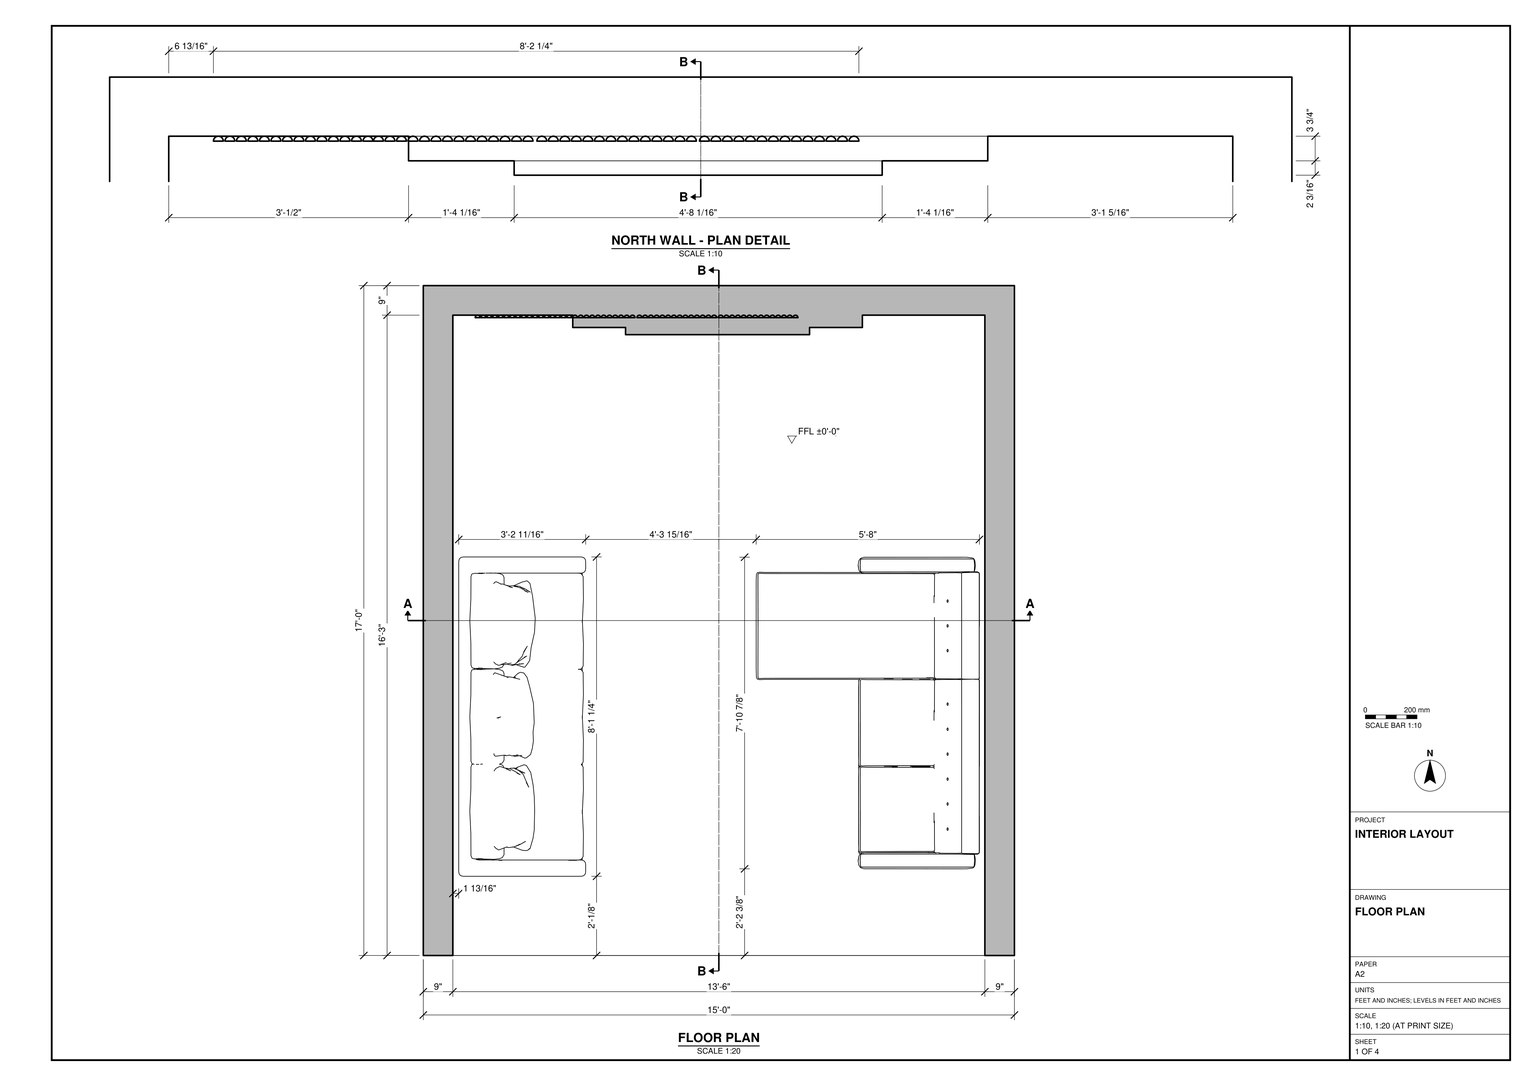
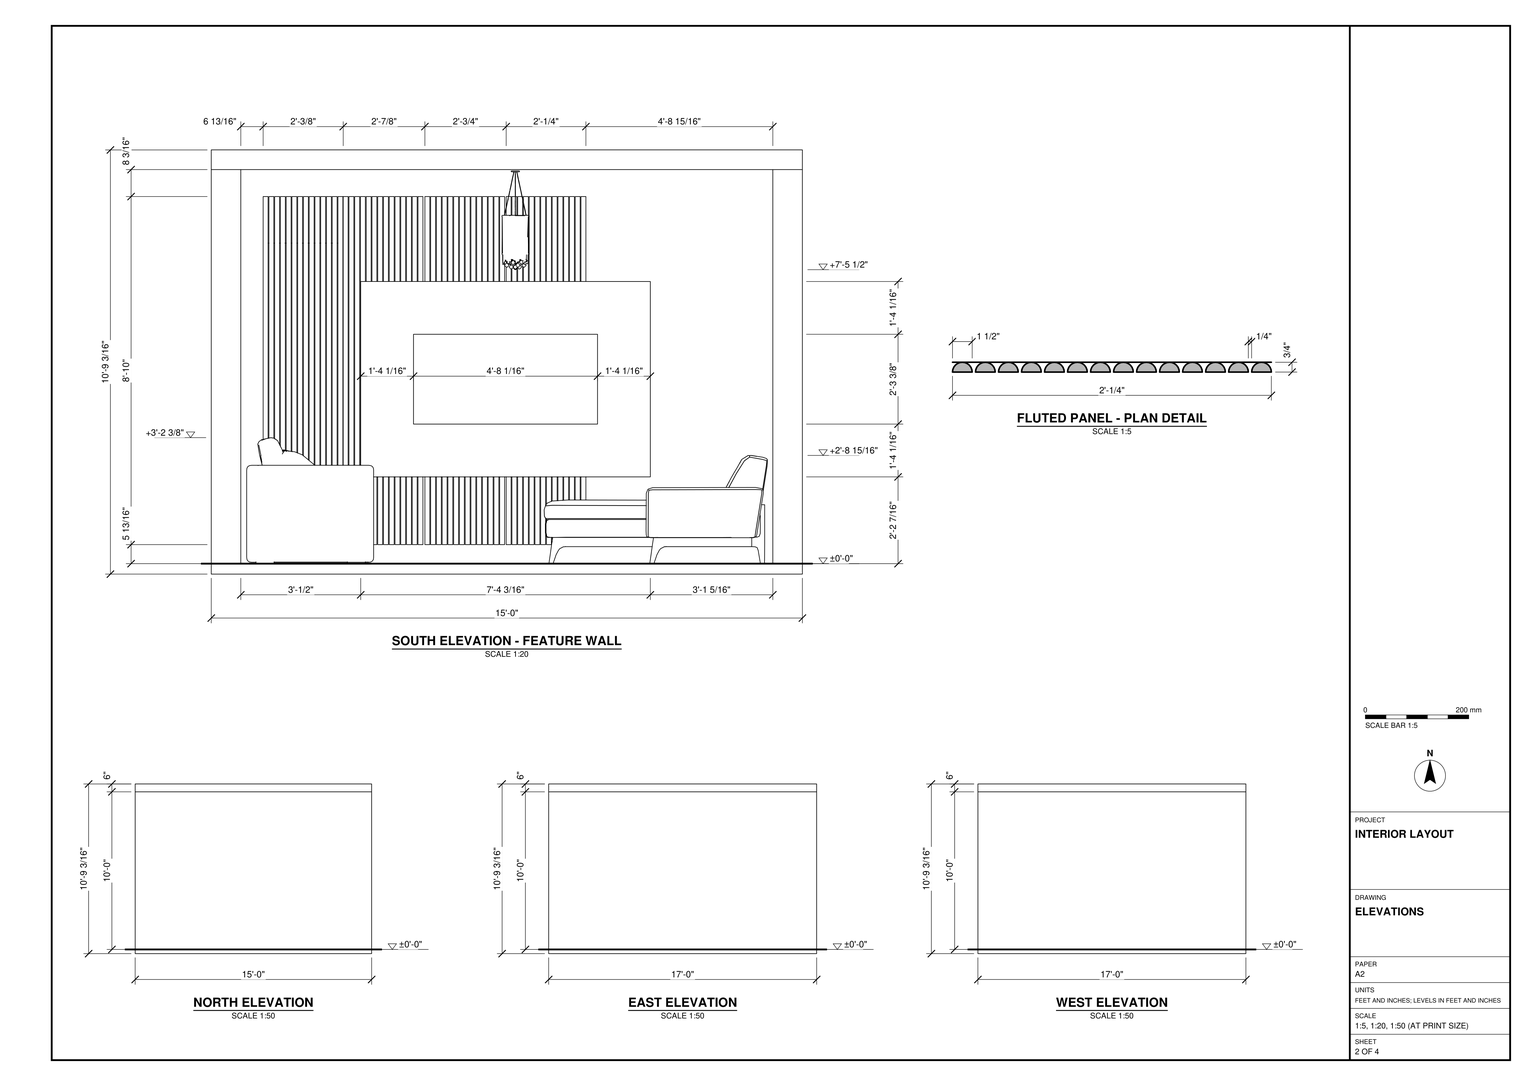
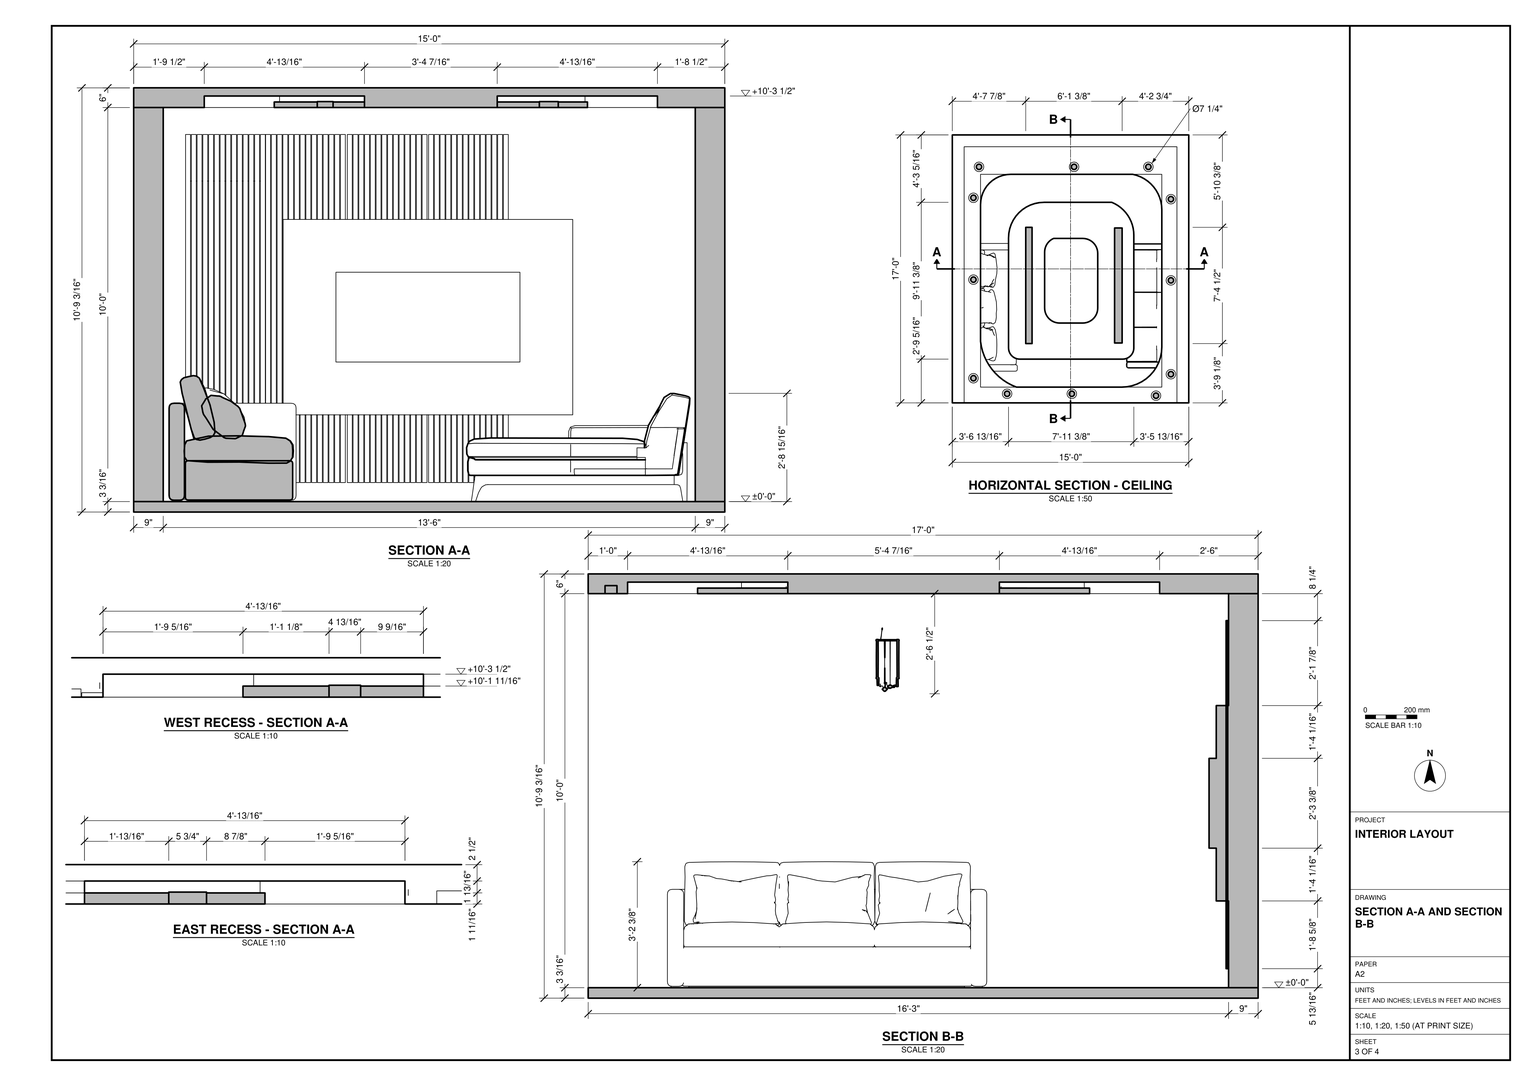
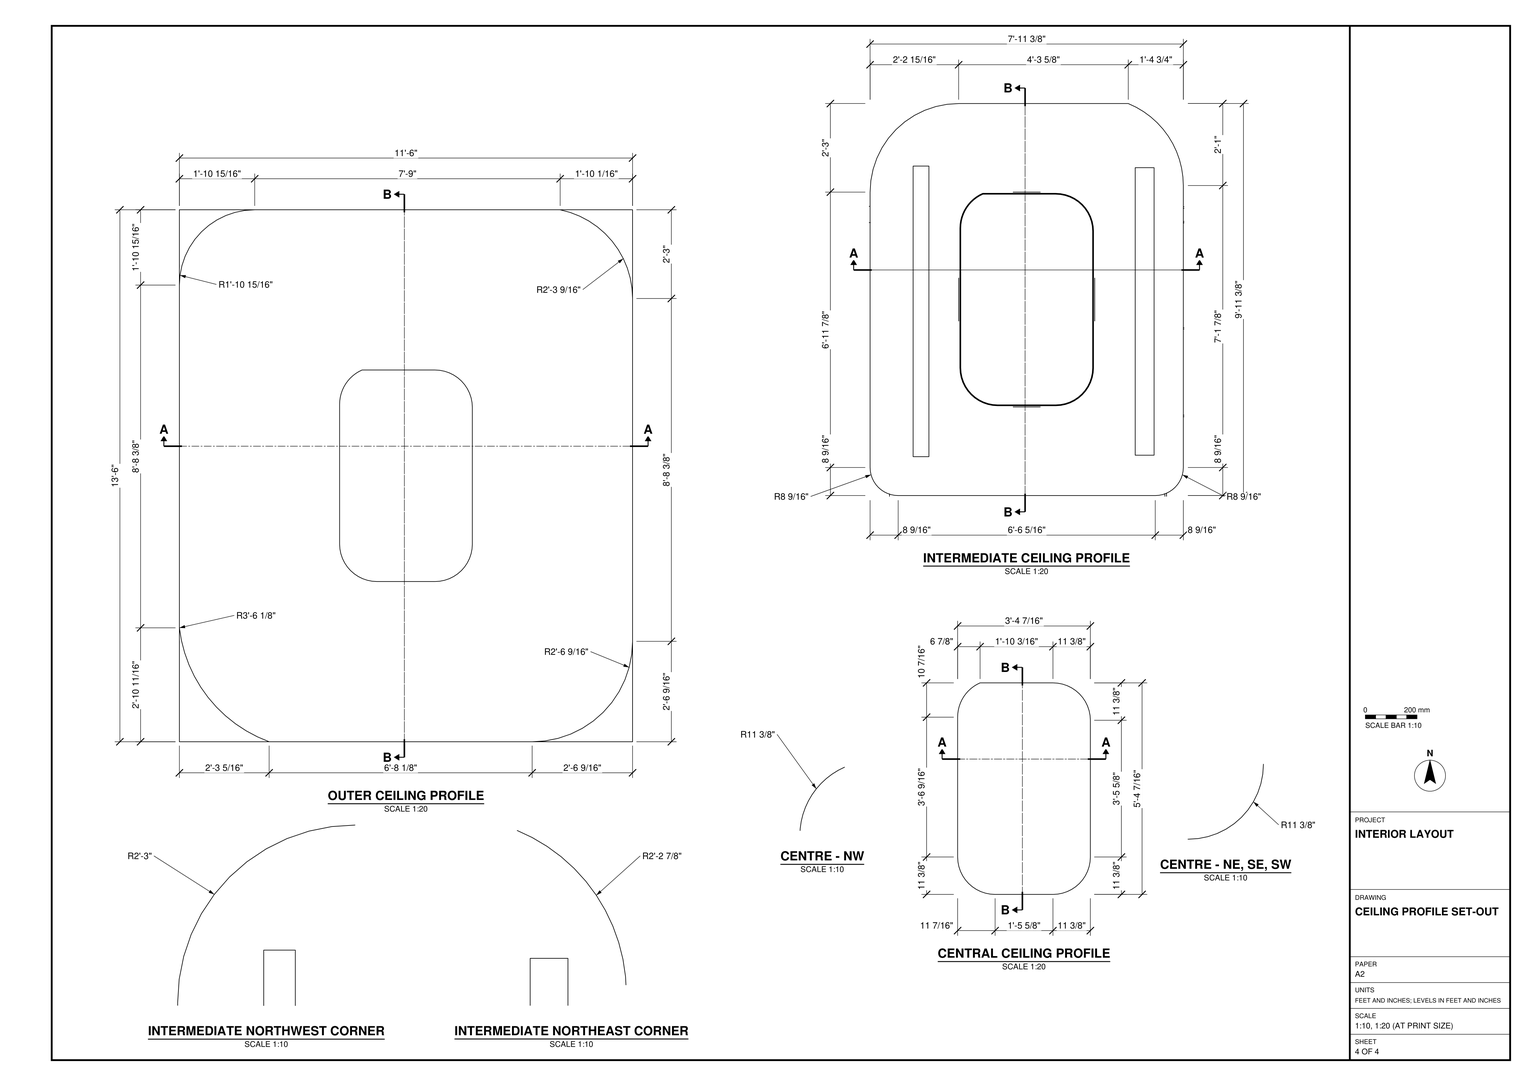
Build the sitting room in SketchUp using task_files/diagram_01.pdf. Work in feet and inches. Set the finished floor level to ±0'-0". The room shell measures 15'-0" east to west and 17'-0" north to south, with an overall height of 10'-9 3/16". Model the floor slab, the 9" north, east and west walls, and the ceiling slab. Leave the south side open as drawn.

Use the north wall plan detail and feature-wall elevation together. Form the vertical flutes with rounded profiles, then place the broad rectangular backing panel in front of them with the television centred on its face. Keep the fluted field offset to the west so it remains visible to the left of the backing panel as well as above and below it. Place the straight sofa along the west wall and the opposing sofa along the east wall, with its chaise projecting into the room at the north end. Match their footprints and setbacks to the floor plan.

Use the horizontal ceiling section for the rounded outlines, paired linear features and perimeter light positions, and the vertical sections for the recess depths and pendant position. Decor and loose items, including lights and cushions, may be any suitable library components. Keep the shell elements and each furniture or joinery piece in separate groups or components, using components for repeated parts. Save one SketchUp model as output_files/sitting_room_with_a_fluted_television_wall.skp.

# SketchUp Ruby script. Lengths in inches.
U = 1.inch
M = Sketchup.active_model
def pt(a) = Geom::Point3d.new(a.map { |v| v * U })
def face(e, loops, mat)
  f = e.add_face(loops[0].map { |a| pt(a) })
  loops[1..].each { |l| e.add_face(l.map { |a| pt(a) }).erase! }
  f.material = f.back_material = mat if mat
  f
end
# faces: each face lists its corners as indices into pts; further lists are holes
def faces(e, pts, list, mat = nil) = list.each { |f| face(e, (f[0].is_a?(Array) ? f : [f]).map { |l| l.map { |i| pts[i] } }, mat) }
# xy, xz, yz: faces in a plane at the given z, y or x. An outline is a flat list of corners, or four numbers for a rectangle; further outlines are holes
def ring(l) = l.size == 4 ? [[l[0], l[1]], [l[2], l[1]], [l[2], l[3]], [l[0], l[3]]] : l.each_slice(2).to_a
def flat(e, list, mat, &to3) = list.each { |f| face(e, (f[0].is_a?(Array) ? f : [f]).map { |l| ring(l).map { |u, v| to3.(u, v) } }, mat) }
def xy(e, z, list, mat = nil) = flat(e, list, mat) { |x, y| [x, y, z] }
def xz(e, y, list, mat = nil) = flat(e, list, mat) { |x, z| [x, y, z] }
def yz(e, x, list, mat = nil) = flat(e, list, mat) { |y, z| [x, y, z] }
def lines(e, pts, list) = list.each { |a, b| e.add_line(pt(pts[a]), pt(pts[b])) }
# prism: a flat outline (further loops are holes) pulled along v
def prism(e, loops, v, mat = nil)
  f = face(e, loops, mat); d = Geom::Vector3d.new(v.map { |x| x * U })
  f.pushpull(f.normal.samedirection?(d) ? d.length : -d.length)
end
def box(e, o, s, mat = nil) = prism(e, [[o, [o[0] + s[0], o[1], o[2]], [o[0] + s[0], o[1] + s[1], o[2]], [o[0], o[1] + s[1], o[2]]]], [0, 0, s[2]], mat)
def at(x, y, z, deg = 0) = Geom::Transformation.translation(pt([x, y, z])) * Geom::Transformation.rotation(ORIGIN, Z_AXIS, deg.degrees)
def axes(o, x, y, z) = Geom::Transformation.new([*x, 0, *y, 0, *z, 0, *pt(o).to_a, 1])
def part(name) = M.definitions.add(name)
# library, detail: a bought-in or finely detailed component or shape, given as its bounding box
def library(name, o, s) = part(name).tap { |d| box(d.entities, o, s) }
def detail(e, o, s) = box(e.add_group.entities, o, s)
def put(e, d, t, mat = nil) = e.add_instance(d, t).tap { |i| i.material = mat if mat }
def group(e, t, mat = nil) = e.add_group.tap { |g| g.transformation = t; g.material = mat if mat }.entities
root = M.entities
M.materials.add("TV").color = [52, 43, 72]
M.materials.add("[Carrera Marble]").color = [207, 207, 207]
M.materials.add("[Translucent Glass Safety]").color = [204, 235, 244]
M.materials["[Translucent Glass Safety]"].alpha = 0.5
M.materials.add("[Translucent Glass Tinted]").color = [8, 201, 241]
M.materials["[Translucent Glass Tinted]"].alpha = 0.48
M.materials.add("[Wood Veneer 01]").color = [120, 70, 37]
c1 = library("Tyler Sofa with Chaise",[-47.45,-33.89,-0.01],[94.9,67.99,32.96])
c2 = library("Sofa 193 003 01",[-48.62,-19.33,0],[97.24,38.66,38.37])
c3 = library("Recessed ceiling lights",[0,0,-4.875],[157.57,181.46,4.875])
c4 = library("Ceiling Lamp 298 001",[-7.99,-7.99,-104.37],[15.97,15.98,104.68])
c5 = library("Group\#6",[-0.5,-0.5,0],[74.38,89.5,1.8125])
c6 = library("Mesh Light\#2",[-0.5,-0.5,-0.1],[1,1,0.2])
c7 = library("Mesh Light\#1",[-0.5,-0.5,-0.1],[1,1,0.2])
c8 = part("SG_Round_Panel")
prism(c8.entities,[[[0.75,0,0],[-0.75,0,0],[-0.72,0.19,0],[-0.65,0.375,0],[-0.53,0.53,0],[-0.375,0.65,0],[-0.19,0.72,0],[0,0.75,0],[0.19,0.72,0],[0.375,0.65,0],[0.53,0.53,0],[0.65,0.375,0],[0.72,0.19,0]]],[0,0,106])
c9 = part("Group20\#1")
put(c9.entities,c8,at(17.02,195,101.6))
put(c9.entities,c8,at(18.77,195,101.6))
put(c9.entities,c8,at(20.52,195,101.6))
put(c9.entities,c8,at(22.27,195,101.6))
put(c9.entities,c8,at(24.02,195,101.6))
put(c9.entities,c8,at(25.77,195,101.6))
put(c9.entities,c8,at(27.53,195,101.6))
put(c9.entities,c8,at(29.28,195,101.6))
put(c9.entities,c8,at(31.03,195,101.6))
put(c9.entities,c8,at(32.78,195,101.6))
put(c9.entities,c8,at(34.53,195,101.6))
put(c9.entities,c8,at(36.29,195,101.6))
put(c9.entities,c8,at(38.04,195,101.6))
put(c9.entities,c8,at(39.79,195,101.6))
put(root,c1,at(135.25,73.84,0,-90))
put(root,c2,at(30.12,72.75,0,90))
g1 = group(root,at(9.49,0,89.51))
xy(g1,30.49,[[[-9.49,0,170.51,204],[12,12,150,174]],[12,12,12,46.6875,12.625,42.86,13.6,39.11,14.91,35.47,16.55,31.96,18.51,28.62,20.76,25.47,23.3,22.55,26.09,19.86,29.12,17.45,32.36,15.32,35.77,13.5,39.35,12],[119.43,12,123.42,12.26,127.34,13.04,131.125,14.33,134.71,16.1,138.04,18.32,141.04,20.96,143.68,23.96,145.9,27.29,147.67,30.875,148.96,34.66,149.74,38.58,150,42.57,150,12],[[41.86,33.3125,40.74,33.38,39.64,33.6,38.59,33.96,37.58,34.46,36.65,35.08,35.8125,35.8125,35.08,36.65,34.46,37.58,33.96,38.59,33.6,39.64,33.38,40.74,33.3125,41.86,33.3125,125.71,33.54,129.23,34.23,132.69,35.36,136.03,36.93,139.2,38.89,142.13,41.21,144.79,43.87,147.11,46.8,149.07,49.97,150.64,53.31,151.77,56.77,152.46,60.29,152.6875,111.92,152.6875,114.33,151.5625,116.61,150.21,118.75,148.63,120.73,146.85,122.52,144.89,124.11,142.76,125.48,140.48,126.62,138.08,127.52,135.58,128.17,133,128.56,130.37,128.6875,127.71,128.6875,41.86,128.62,40.74,128.4,39.64,128.04,38.59,127.54,37.58,126.92,36.65,126.1875,35.8125,125.35,35.08,124.42,34.46,123.41,33.96,122.36,33.6,121.26,33.38,120.14,33.3125],[72.19,60.79,89.81,60.79,91.3,60.89,92.76,61.18,94.18,61.66,95.51,62.32,96.42,62.92,96.75,63.14,97.875,64.125,98.86,65.25,99.68,66.49,100.34,67.82,100.82,69.24,101.11,70.7,101.21,72.19,101.21,113.81,101.11,115.3,100.82,116.76,100.34,118.18,99.68,119.51,98.86,120.75,97.875,121.875,96.75,122.86,95.51,123.68,94.18,124.34,92.76,124.82,91.3,125.11,89.81,125.21,67.62,125.21,66.63,124.72,65.7,124.14,64.83,123.47,64.02,122.72,63.29,121.9,62.65,121.01,62.09,120.06,61.63,119.0625,61.26,118.02,61,116.96,60.84,115.87,60.79,114.77,60.79,72.19,60.89,70.7,61.18,69.24,61.66,67.82,62.32,66.49,63.14,65.25,64.125,64.125,65.25,63.14,65.58,62.92,66.49,62.32,67.82,61.66,69.24,61.18,70.7,60.89],[114.04,45.6,119.79,133.16],[46.41,45.15,51.23,133.65]],[150,146.98,149.82,150.12,149.29,153.22,148.4,156.24,147.18,159.13,145.63,161.875,143.79,164.42,141.66,166.74,139.29,168.8,136.69,170.58,133.91,172.05,130.98,173.2,127.94,174,150,174],
  [12,151.0625,12,174,34.9375,174,31.94,173.8,29,173.22,26.16,172.25,23.47,170.93,20.97,169.26,18.72,167.28,16.74,165.03,15.07,162.53,13.75,159.84,12.78,157,12.2,154.06]])
xy(g1,30.49,[[72.19,60.79,70.7,60.89,69.24,61.18,67.82,61.66,66.49,62.32,65.58,62.92,65.25,63.14,64.125,64.125,63.14,65.25,62.32,66.49,61.66,67.82,61.18,69.24,60.89,70.7,60.79,72.19,60.79,114.77,60.84,115.87,61,116.96,61.26,118.02,61.63,119.0625,62.09,120.06,62.65,121.01,63.29,121.9,64.02,122.72,64.83,123.47,65.7,124.14,66.63,124.72,67.62,125.21,89.81,125.21,91.3,125.11,92.76,124.82,94.18,124.34,95.51,123.68,96.75,122.86,97.875,121.875,98.86,120.75,99.68,119.51,100.34,118.18,100.82,116.76,101.11,115.3,101.21,113.81,101.21,72.19,101.11,70.7,100.82,69.24,100.34,67.82,99.68,66.49,98.86,65.25,97.875,64.125,96.75,63.14,96.42,62.92,95.51,62.32,94.18,61.66,92.76,61.18,91.3,60.89,89.81,60.79]],"[Translucent Glass Safety]")
xy(g1,30.49,[[46.41,45.15,51.23,133.65],[114.04,45.6,119.79,133.16]],"[Translucent Glass Tinted]")
xy(g1,32.18,[[[41.86,33.3125,120.14,33.3125,121.26,33.38,122.36,33.6,123.41,33.96,124.42,34.46,125.35,35.08,126.1875,35.8125,126.92,36.65,127.54,37.58,128.04,38.59,128.4,39.64,128.62,40.74,128.6875,41.86,128.6875,127.71,128.56,130.37,128.17,133,127.52,135.58,126.62,138.08,125.48,140.48,124.11,142.76,122.52,144.89,120.73,146.85,118.75,148.63,116.61,150.21,114.33,151.5625,111.92,152.6875,60.29,152.6875,56.77,152.46,53.31,151.77,49.97,150.64,46.8,149.07,43.87,147.11,41.21,144.79,38.89,142.13,36.93,139.2,35.36,136.03,34.23,132.69,33.54,129.23,33.3125,125.71,33.3125,41.86,33.38,40.74,33.6,39.64,33.96,38.59,34.46,37.58,35.08,36.65,35.8125,35.8125,36.65,35.08,37.58,34.46,38.59,33.96,39.64,33.6,40.74,33.38],[72.19,60.79,70.7,60.89,69.24,61.18,67.82,61.66,66.49,62.32,65.58,62.92,65.25,63.14,64.125,64.125,63.14,65.25,62.32,66.49,61.66,67.82,61.18,69.24,60.89,70.7,60.79,72.19,60.79,114.77,60.84,115.87,61,116.96,61.26,118.02,61.63,119.0625,62.09,120.06,62.65,121.01,63.29,121.9,64.02,122.72,64.83,123.47,65.7,124.14,66.63,124.72,67.62,125.21,89.81,125.21,91.3,125.11,92.76,124.82,94.18,124.34,95.51,123.68,96.75,122.86,97.875,121.875,98.86,120.75,99.68,119.51,100.34,118.18,100.82,116.76,101.11,115.3,101.21,113.81,101.21,72.19,101.11,70.7,100.82,69.24,100.34,67.82,99.68,66.49,98.86,65.25,97.875,64.125,96.75,63.14,96.42,62.92,95.51,62.32,94.18,61.66,92.76,61.18,91.3,60.89,89.81,60.79],[114.04,45.6,119.79,133.16],[46.41,45.15,51.23,133.65]]])
xy(g1,33.99,[[[39.35,12,35.77,13.5,32.36,15.32,29.12,17.45,26.09,19.86,23.3,22.55,20.76,25.47,18.51,28.62,16.55,31.96,14.91,35.47,13.6,39.11,12.625,42.86,12,46.6875,12,151.0625,12.2,154.06,12.78,157,13.75,159.84,15.07,162.53,16.74,165.03,18.72,167.28,20.97,169.26,23.47,170.93,26.16,172.25,29,173.22,31.94,173.8,34.9375,174,127.94,174,130.98,173.2,133.91,172.05,136.69,170.58,139.29,168.8,141.66,166.74,143.79,164.42,145.63,161.875,147.18,159.13,148.4,156.24,149.29,153.22,149.82,150.12,150,146.98,150,42.57,149.74,38.58,148.96,34.66,147.67,30.875,145.9,27.29,143.68,23.96,141.04,20.96,138.04,18.32,134.71,16.1,131.125,14.33,127.34,13.04,123.42,12.26,119.43,12],[72.19,60.79,89.81,60.79,91.3,60.89,92.76,61.18,94.18,61.66,95.51,62.32,96.75,63.14,97.875,64.125,98.86,65.25,99.68,66.49,100.34,67.82,100.82,69.24,101.11,70.7,101.21,72.19,101.21,113.81,101.11,115.3,100.82,116.76,100.34,118.18,99.68,119.51,98.86,120.75,97.875,121.875,96.75,122.86,95.51,123.68,94.18,124.34,92.76,124.82,91.3,125.11,89.81,125.21,67.62,125.21,66.63,124.72,65.7,124.14,64.83,123.47,64.02,122.72,63.29,121.9,62.65,121.01,62.09,120.06,61.63,119.0625,61.26,118.02,61,116.96,60.84,115.87,60.79,114.77,60.79,72.19,60.89,70.7,61.18,69.24,61.66,67.82,62.32,66.49,63.14,65.25,64.125,64.125,65.25,63.14,66.49,62.32,67.82,61.66,69.24,61.18,70.7,60.89]]])
xy(g1,36.49,[[-9.49,0,170.51,204]])
xz(g1,0,[[-9.49,30.49,170.51,36.49]])
xz(g1,33.3125,[[41.86,30.49,120.14,32.18]])
xz(g1,45.15,[[46.41,30.49,51.23,32.18]])
xz(g1,45.6,[[114.04,30.49,119.79,32.18]])
xz(g1,60.79,[[72.19,30.49,89.81,32.18]])
xz(g1,125.21,[[67.62,30.49,89.81,32.18]])
xz(g1,133.16,[[114.04,30.49,119.79,32.18]])
xz(g1,133.65,[[46.41,30.49,51.23,32.18],[46.41,32.18,51.23,32.3]])
xz(g1,152.6875,[[60.29,30.49,111.92,32.18]])
xz(g1,204,[[-9.49,30.49,170.51,36.49]])
yz(g1,-9.49,[[0,30.49,204,36.49]])
yz(g1,33.3125,[[41.86,30.49,125.71,32.18]])
yz(g1,46.41,[[45.15,30.49,133.65,32.18]])
yz(g1,51.23,[[45.15,30.49,133.65,32.18]])
yz(g1,60.79,[[72.19,30.49,114.77,32.18]])
yz(g1,101.21,[[72.19,30.49,113.81,32.18]])
yz(g1,114.04,[[45.6,30.49,133.16,32.18]])
yz(g1,119.79,[[45.6,30.49,133.16,32.18]])
yz(g1,128.6875,[[41.86,30.49,127.71,32.18]])
yz(g1,170.51,[[0,30.49,204,36.49]])
p = [[40.74,33.38,30.49],[41.86,33.3125,30.49],[41.86,33.3125,32.18],[40.74,33.38,32.18],[120.14,33.3125,30.49],[121.26,33.38,30.49],
  [121.26,33.38,32.18],[120.14,33.3125,32.18],[39.64,33.6,30.49],[39.64,33.6,32.18],[122.36,33.6,30.49],[122.36,33.6,32.18],
  [38.59,33.96,30.49],[38.59,33.96,32.18],[123.41,33.96,30.49],[123.41,33.96,32.18],[37.58,34.46,30.49],[37.58,34.46,32.18],
  [124.42,34.46,30.49],[124.42,34.46,32.18],[36.65,35.08,30.49],[36.65,35.08,32.18],[125.35,35.08,30.49],[125.35,35.08,32.18],
  [35.8125,35.8125,30.49],[35.8125,35.8125,32.18],[126.1875,35.8125,30.49],[126.1875,35.8125,32.18],[35.08,36.65,30.49],[35.08,36.65,32.18],
  [126.92,36.65,30.49],[126.92,36.65,32.18],[34.46,37.58,30.49],[34.46,37.58,32.18],[127.54,37.58,30.49],[127.54,37.58,32.18],
  [33.96,38.59,30.49],[33.96,38.59,32.18],[128.04,38.59,30.49],[128.04,38.59,32.18],[33.6,39.64,30.49],[33.6,39.64,32.18],
  [128.4,39.64,30.49],[128.4,39.64,32.18],[33.38,40.74,30.49],[33.38,40.74,32.18],[128.62,40.74,30.49],[128.62,40.74,32.18],
  [33.3125,41.86,30.49],[33.3125,41.86,32.18],[128.6875,41.86,30.49],[128.6875,41.86,32.18],[72.19,60.79,30.49],[70.7,60.89,30.49],
  [70.7,60.89,32.18],[72.19,60.79,32.18],[91.3,60.89,30.49],[89.81,60.79,30.49],[89.81,60.79,32.18],[91.3,60.89,32.18],
  [69.24,61.18,30.49],[69.24,61.18,32.18],[92.76,61.18,30.49],[92.76,61.18,32.18],[67.82,61.66,30.49],[67.82,61.66,32.18],
  [94.18,61.66,30.49],[94.18,61.66,32.18],[66.49,62.32,30.49],[66.49,62.32,32.18],[95.51,62.32,30.49],[95.51,62.32,32.18],
  [65.58,62.92,30.49],[65.58,62.92,32.18],[96.42,62.92,30.49],[96.42,62.92,32.18],[65.25,63.14,30.49],[65.25,63.14,32.18],
  [96.75,63.14,30.49],[96.75,63.14,32.18],[64.125,64.125,30.49],[64.125,64.125,32.18],[97.875,64.125,30.49],[97.875,64.125,32.18],
  [63.14,65.25,30.49],[63.14,65.25,32.18],[98.86,65.25,30.49],[98.86,65.25,32.18],[62.32,66.49,30.49],[62.32,66.49,32.18],
  [99.68,66.49,30.49],[99.68,66.49,32.18],[61.66,67.82,30.49],[61.66,67.82,32.18],[100.34,67.82,30.49],[100.34,67.82,32.18],
  [61.18,69.24,30.49],[61.18,69.24,32.18],[100.82,69.24,30.49],[100.82,69.24,32.18],[60.89,70.7,30.49],[60.89,70.7,32.18],
  [101.11,70.7,30.49],[101.11,70.7,32.18],[60.79,72.19,30.49],[60.79,72.19,32.18],[101.21,72.19,30.49],[101.21,72.19,32.18],
  [101.11,115.3,30.49],[101.21,113.81,30.49],[101.21,113.81,32.18],[101.11,115.3,32.18],[60.79,114.77,30.49],[60.84,115.87,30.49],
  [60.84,115.87,32.18],[60.79,114.77,32.18],[100.82,116.76,30.49],[100.82,116.76,32.18],[61,116.96,30.49],[61,116.96,32.18],
  [100.34,118.18,30.49],[100.34,118.18,32.18],[61.26,118.02,30.49],[61.26,118.02,32.18],[61.63,119.0625,30.49],[61.63,119.0625,32.18],
  [99.68,119.51,30.49],[99.68,119.51,32.18],[62.09,120.06,30.49],[62.09,120.06,32.18],[98.86,120.75,30.49],[98.86,120.75,32.18],
  [62.65,121.01,30.49],[62.65,121.01,32.18],[97.875,121.875,30.49],[97.875,121.875,32.18],[63.29,121.9,30.49],[63.29,121.9,32.18],
  [64.02,122.72,30.49],[64.02,122.72,32.18],[96.75,122.86,30.49],[96.75,122.86,32.18],[64.83,123.47,30.49],[64.83,123.47,32.18],
  [95.51,123.68,30.49],[95.51,123.68,32.18],[65.7,124.14,30.49],[65.7,124.14,32.18],[94.18,124.34,30.49],[94.18,124.34,32.18],
  [66.63,124.72,30.49],[66.63,124.72,32.18],[92.76,124.82,30.49],[92.76,124.82,32.18],[67.62,125.21,30.49],[67.62,125.21,32.18],
  [91.3,125.11,30.49],[91.3,125.11,32.18],[89.81,125.21,30.49],[89.81,125.21,32.18],[33.54,129.23,30.49],[33.3125,125.71,30.49],
  [33.3125,125.71,32.18],[33.54,129.23,32.18],[128.6875,127.71,30.49],[128.56,130.37,30.49],[128.56,130.37,32.18],[128.6875,127.71,32.18],
  [34.23,132.69,30.49],[34.23,132.69,32.18],[128.17,133,30.49],[128.17,133,32.18],[35.36,136.03,30.49],[35.36,136.03,32.18],
  [127.52,135.58,30.49],[127.52,135.58,32.18],[126.62,138.08,30.49],[126.62,138.08,32.18],[36.93,139.2,30.49],[36.93,139.2,32.18],
  [125.48,140.48,30.49],[125.48,140.48,32.18],[38.89,142.13,30.49],[38.89,142.13,32.18],[124.11,142.76,30.49],[124.11,142.76,32.18],
  [41.21,144.79,30.49],[41.21,144.79,32.18],[122.52,144.89,30.49],[122.52,144.89,32.18],[43.87,147.11,30.49],[43.87,147.11,32.18],
  [120.73,146.85,30.49],[120.73,146.85,32.18],[118.75,148.63,30.49],[118.75,148.63,32.18],[46.8,149.07,30.49],[46.8,149.07,32.18],
  [116.61,150.21,30.49],[116.61,150.21,32.18],[49.97,150.64,30.49],[49.97,150.64,32.18],[114.33,151.5625,30.49],[114.33,151.5625,32.18],
  [53.31,151.77,30.49],[53.31,151.77,32.18],[111.92,152.6875,30.49],[111.92,152.6875,32.18],[56.77,152.46,30.49],[56.77,152.46,32.18],
  [60.29,152.6875,30.49],[60.29,152.6875,32.18]]
faces(g1,p,[[0,1,2,3],[4,5,6,7],[8,0,3,9],[5,10,11,6],[12,8,9,13],[10,14,15,11],[16,12,13,17],[14,18,19,15],
  [20,16,17,21],[18,22,23,19],[24,20,21,25],[22,26,27,23],[28,24,25,29],[26,30,31,27],[32,28,29,33],[30,34,35,31],
  [36,32,33,37],[34,38,39,35],[40,36,37,41],[38,42,43,39],[44,40,41,45],[42,46,47,43],[48,44,45,49],[46,50,51,47],
  [52,53,54,55],[56,57,58,59],[53,60,61,54],[62,56,59,63],[60,64,65,61],[66,62,63,67],[64,68,69,65],[70,66,67,71],
  [68,72,73,69],[74,70,71,75],[72,76,77,73],[78,74,75,79],[76,80,81,77],[82,78,79,83],[80,84,85,81],[86,82,83,87],
  [84,88,89,85],[90,86,87,91],[88,92,93,89],[94,90,91,95],[92,96,97,93],[98,94,95,99],[96,100,101,97],[102,98,99,103],
  [100,104,105,101],[106,102,103,107],[108,109,110,111],[112,113,114,115],[116,108,111,117],[113,118,119,114],[120,116,117,121],[118,122,123,119],
  [122,124,125,123],[126,120,121,127],[124,128,129,125],[130,126,127,131],[128,132,133,129],[134,130,131,135],[132,136,137,133],[136,138,139,137],
  [140,134,135,141],[138,142,143,139],[144,140,141,145],[142,146,147,143],[148,144,145,149],[146,150,151,147],[152,148,149,153],[150,154,155,151],
  [156,152,153,157],[158,156,157,159],[160,161,162,163],[164,165,166,167],[168,160,163,169],[165,170,171,166],[172,168,169,173],[170,174,175,171],
  [174,176,177,175],[178,172,173,179],[176,180,181,177],[182,178,179,183],[180,184,185,181],[186,182,183,187],[184,188,189,185],[190,186,187,191],
  [188,192,193,189],[192,194,195,193],[196,190,191,197],[194,198,199,195],[200,196,197,201],[198,202,203,199],[204,200,201,205],[202,206,207,203],
  [208,204,205,209],[210,208,209,211]])
put(g1,c3,axes([160.53,1.88,30.49],[-1,0,0],[0,1,0],[0,0,-1]))
put(g1,c4,axes([83.1,91.17,30.01],[0.51197,0,0],[0,0.5724,0],[0,0,0.28752]))
put(g1,c5,at(46.41,45.15,30.49))
g2 = group(g1,at(12,12,30.49))
xz(g2,0,[[27.35,0,107.43,3.5]])
xz(g2,162,[[22.9375,0,115.94,3.5]])
yz(g2,0,[[34.6875,0,139.0625,3.5]])
yz(g2,138,[[30.57,0,134.98,3.5]])
p = [[27.35,0,0],[23.77,1.5,0],[23.77,1.5,3.5],[27.35,0,3.5],[111.42,0.26,0],[107.43,0,0],
  [107.43,0,3.5],[111.42,0.26,3.5],[115.34,1.04,0],[115.34,1.04,3.5],[119.125,2.33,0],[119.125,2.33,3.5],
  [20.36,3.32,0],[20.36,3.32,3.5],[122.71,4.1,0],[122.71,4.1,3.5],[17.12,5.45,0],[17.12,5.45,3.5],
  [126.04,6.32,0],[126.04,6.32,3.5],[14.09,7.86,0],[14.09,7.86,3.5],[129.04,8.96,0],[129.04,8.96,3.5],
  [11.3,10.55,0],[11.3,10.55,3.5],[131.68,11.96,0],[131.68,11.96,3.5],[8.76,13.47,0],[8.76,13.47,3.5],
  [133.9,15.29,0],[133.9,15.29,3.5],[6.51,16.62,0],[6.51,16.62,3.5],[135.67,18.875,0],[135.67,18.875,3.5],
  [4.55,19.96,0],[4.55,19.96,3.5],[136.96,22.66,0],[136.96,22.66,3.5],[2.91,23.47,0],[2.91,23.47,3.5],
  [137.74,26.58,0],[137.74,26.58,3.5],[1.6,27.11,0],[1.6,27.11,3.5],[138,30.57,0],[138,30.57,3.5],
  [0.625,30.86,0],[0.625,30.86,3.5],[0,34.6875,0],[0,34.6875,3.5],[137.82,138.12,0],[138,134.98,0],
  [138,134.98,3.5],[137.82,138.12,3.5],[137.29,141.22,0],[137.29,141.22,3.5],[0,139.0625,0],[0.2,142.06,0],
  [0.2,142.06,3.5],[0,139.0625,3.5],[136.4,144.24,0],[136.4,144.24,3.5],[0.78,145,0],[0.78,145,3.5],
  [135.18,147.13,0],[135.18,147.13,3.5],[1.75,147.84,0],[1.75,147.84,3.5],[133.63,149.875,0],[133.63,149.875,3.5],
  [3.07,150.53,0],[3.07,150.53,3.5],[131.79,152.42,0],[131.79,152.42,3.5],[4.74,153.03,0],[4.74,153.03,3.5],
  [129.66,154.74,0],[129.66,154.74,3.5],[6.72,155.28,0],[6.72,155.28,3.5],[127.29,156.8,0],[127.29,156.8,3.5],
  [8.97,157.26,0],[8.97,157.26,3.5],[124.69,158.58,0],[124.69,158.58,3.5],[11.47,158.93,0],[11.47,158.93,3.5],
  [121.91,160.05,0],[121.91,160.05,3.5],[14.16,160.25,0],[14.16,160.25,3.5],[118.98,161.2,0],[118.98,161.2,3.5],
  [17,161.22,0],[17,161.22,3.5],[19.94,161.8,0],[19.94,161.8,3.5],[115.94,162,0],[115.94,162,3.5],
  [22.9375,162,0],[22.9375,162,3.5]]
faces(g2,p,[[0,1,2,3],[4,5,6,7],[8,4,7,9],[10,8,9,11],[1,12,13,2],[14,10,11,15],[12,16,17,13],[18,14,15,19],
  [16,20,21,17],[22,18,19,23],[20,24,25,21],[26,22,23,27],[24,28,29,25],[30,26,27,31],[28,32,33,29],[34,30,31,35],
  [32,36,37,33],[38,34,35,39],[36,40,41,37],[42,38,39,43],[40,44,45,41],[46,42,43,47],[44,48,49,45],[48,50,51,49],
  [52,53,54,55],[56,52,55,57],[58,59,60,61],[62,56,57,63],[59,64,65,60],[66,62,63,67],[64,68,69,65],[70,66,67,71],
  [68,72,73,69],[74,70,71,75],[72,76,77,73],[78,74,75,79],[76,80,81,77],[82,78,79,83],[80,84,85,81],[86,82,83,87],
  [84,88,89,85],[90,86,87,91],[88,92,93,89],[94,90,91,95],[92,96,97,93],[96,98,99,97],[100,94,95,101],[98,102,103,99]])
put(g2,c6,axes([69,81,1.75],[139,0,0],[0,163,0],[0,0,4.5]))
g3 = group(g1,at(60.79,60.79,30.49))
xz(g3,0,[[11.4,0,29.03,3.5]])
xz(g3,64.42,[[6.83,0,29.03,3.5]])
yz(g3,0,[[11.4,0,53.98,3.5]])
yz(g3,40.42,[[11.4,0,53.03,3.5]])
p = [[11.4,0,0],[9.91,0.1,0],[9.91,0.1,3.5],[11.4,0,3.5],[30.51,0.1,0],[29.03,0,0],
  [29.03,0,3.5],[30.51,0.1,3.5],[8.45,0.39,0],[8.45,0.39,3.5],[31.98,0.39,0],[31.98,0.39,3.5],
  [7.04,0.87,0],[7.04,0.87,3.5],[33.39,0.87,0],[33.39,0.87,3.5],[5.7,1.53,0],[5.7,1.53,3.5],
  [34.72,1.53,0],[34.72,1.53,3.5],[4.46,2.35,0],[4.46,2.35,3.5],[35.96,2.35,0],[35.96,2.35,3.5],
  [3.34,3.34,0],[3.34,3.34,3.5],[37.08,3.34,0],[37.08,3.34,3.5],[2.35,4.46,0],[2.35,4.46,3.5],
  [38.07,4.46,0],[38.07,4.46,3.5],[1.53,5.7,0],[1.53,5.7,3.5],[38.9,5.7,0],[38.9,5.7,3.5],
  [0.87,7.04,0],[0.87,7.04,3.5],[39.55,7.04,0],[39.55,7.04,3.5],[0.39,8.45,0],[0.39,8.45,3.5],
  [40.03,8.45,0],[40.03,8.45,3.5],[0.1,9.91,0],[0.1,9.91,3.5],[40.32,9.91,0],[40.32,9.91,3.5],
  [0,11.4,0],[0,11.4,3.5],[40.42,11.4,0],[40.42,11.4,3.5],[40.32,54.51,0],[40.42,53.03,0],
  [40.42,53.03,3.5],[40.32,54.51,3.5],[0,53.98,0],[0.05,55.08,0],[0.05,55.08,3.5],[0,53.98,3.5],
  [40.03,55.98,0],[40.03,55.98,3.5],[0.21,56.17,0],[0.21,56.17,3.5],[39.55,57.39,0],[39.55,57.39,3.5],
  [0.47,57.24,0],[0.47,57.24,3.5],[0.84,58.27,0],[0.84,58.27,3.5],[38.9,58.72,0],[38.9,58.72,3.5],
  [1.3,59.27,0],[1.3,59.27,3.5],[38.07,59.96,0],[38.07,59.96,3.5],[1.86,60.22,0],[1.86,60.22,3.5],
  [37.08,61.08,0],[37.08,61.08,3.5],[2.51,61.11,0],[2.51,61.11,3.5],[3.23,61.93,0],[3.23,61.93,3.5],
  [35.96,62.07,0],[35.96,62.07,3.5],[4.04,62.68,0],[4.04,62.68,3.5],[34.72,62.9,0],[34.72,62.9,3.5],
  [4.91,63.35,0],[4.91,63.35,3.5],[33.39,63.55,0],[33.39,63.55,3.5],[5.85,63.93,0],[5.85,63.93,3.5],
  [31.98,64.03,0],[31.98,64.03,3.5],[6.83,64.42,0],[6.83,64.42,3.5],[30.51,64.32,0],[30.51,64.32,3.5],
  [29.03,64.42,0],[29.03,64.42,3.5]]
faces(g3,p,[[0,1,2,3],[4,5,6,7],[1,8,9,2],[10,4,7,11],[8,12,13,9],[14,10,11,15],[12,16,17,13],[18,14,15,19],
  [16,20,21,17],[22,18,19,23],[20,24,25,21],[26,22,23,27],[24,28,29,25],[30,26,27,31],[28,32,33,29],[34,30,31,35],
  [32,36,37,33],[38,34,35,39],[36,40,41,37],[42,38,39,43],[40,44,45,41],[46,42,43,47],[44,48,49,45],[50,46,47,51],
  [52,53,54,55],[56,57,58,59],[60,52,55,61],[57,62,63,58],[64,60,61,65],[62,66,67,63],[66,68,69,67],[70,64,65,71],
  [68,72,73,69],[74,70,71,75],[72,76,77,73],[78,74,75,79],[76,80,81,77],[80,82,83,81],[84,78,79,85],[82,86,87,83],
  [88,84,85,89],[86,90,91,87],[92,88,89,93],[90,94,95,91],[96,92,93,97],[94,98,99,95],[100,96,97,101],[102,100,101,103]])
put(g3,c7,axes([20.21,32.21,1.75],[41.42205,0,0],[0,65.42205,0],[0,0,4.5]))
g4 = group(root,at(0,0,0))
xy(g4,26.42,[[45.51,191.25,133.7,195]])
xy(g4,85.92,[[45.51,191.25,133.7,195]])
xy(g4,120,[[0,0,9,0,9,195,171,195,171,0,180,0,180,204,0,204]])
xz(g4,0,[[0,0,9,120],[171,0,180,120]])
xz(g4,195,[[[9,0,171,120],[45.51,26.42,133.7,85.92],[16.27,5.79,40.08,97.6]],[16.27,5.79,40.08,97.6]])
xz(g4,204,[[0,0,180,120]])
yz(g4,0,[[0,0,204,120]])
yz(g4,9,[[0,0,195,120]])
yz(g4,45.51,[[191.25,26.42,195,85.92]])
yz(g4,133.7,[[191.25,26.42,195,85.92]])
yz(g4,171,[[0,0,195,120]])
yz(g4,180,[[0,0,204,120]])
g5 = group(g4,at(45.51,191.25,26.42),"[Carrera Marble]")
xz(g5,0,[[[0,0,88.1875,59.5],[16.08,16.08,72.11,43.42]]])
g6 = group(g4,at(61.59,189.0625,42.49),"TV")
xy(g6,0,[[0,0,56.03,2.1875]],"TV")
xy(g6,27.35,[[0,0,56.03,2.1875]],"TV")
xz(g6,0,[[0,0,56.03,27.35]],"TV")
yz(g6,0,[[0,0,2.1875,27.35]],"TV")
yz(g6,56.03,[[0,0,2.1875,27.35]],"TV")
put(g4,c9,at(-0.46,-0.75,-95.8125),"[Wood Veneer 01]")
put(g4,c9,at(23.91,-0.75,-95.8125),"[Wood Veneer 01]")
put(g4,c9,at(48.79,-0.75,-95.8125),"[Wood Veneer 01]")
put(g4,c9,at(73.54,-0.75,-95.8125),"[Wood Veneer 01]")
g7 = group(root,at(0,0,-3.1875))
box(g7,[0,0,0],[180,204,3.1875])
